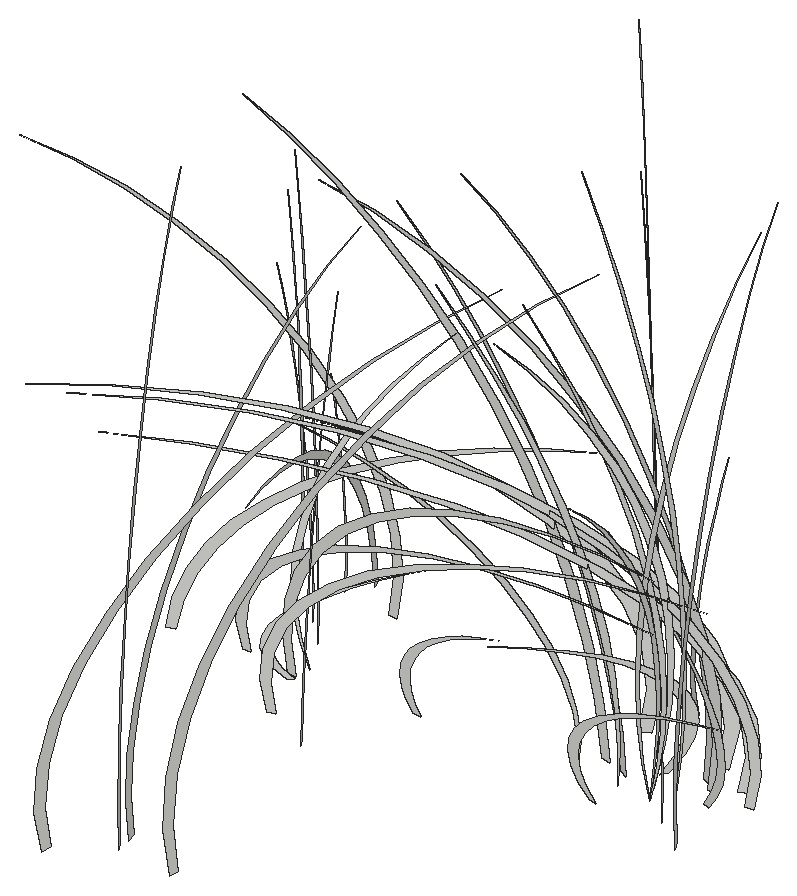
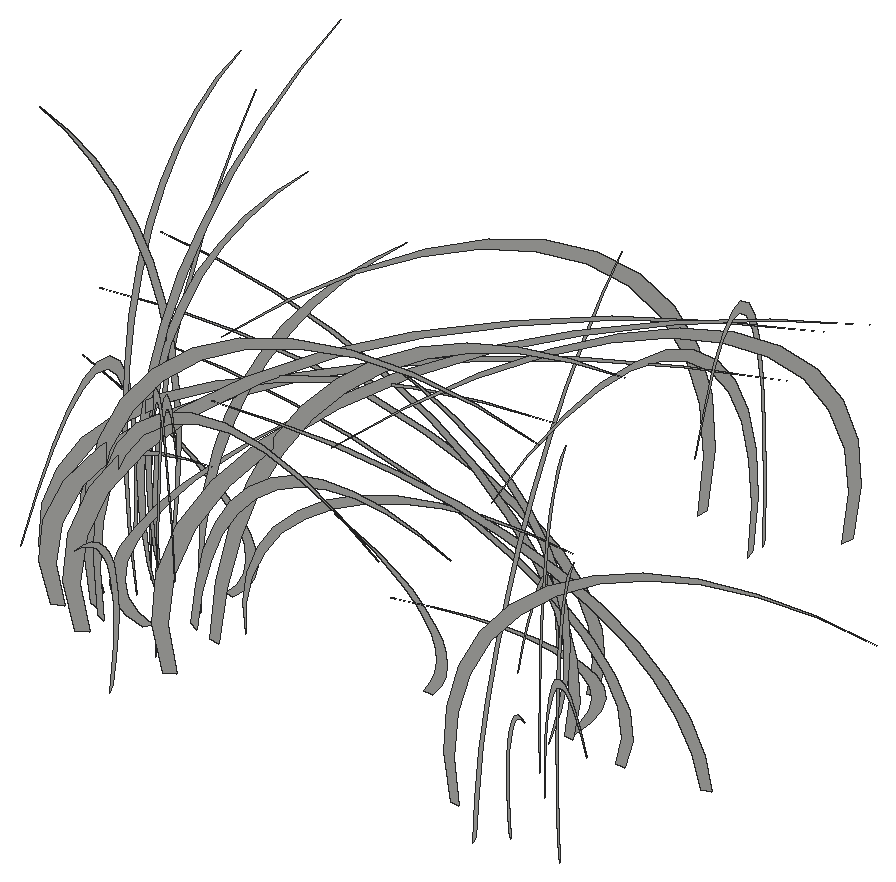
# SketchUp Ruby script. Lengths in inches.
U = 1.inch
M = Sketchup.active_model
def pt(a) = Geom::Point3d.new(a.map { |v| v * U })
def face(e, loops, mat)
  f = e.add_face(loops[0].map { |a| pt(a) })
  loops[1..].each { |l| e.add_face(l.map { |a| pt(a) }).erase! }
  f.material = f.back_material = mat if mat
  f
end
# faces: each face lists its corners as indices into pts; further lists are holes
def faces(e, pts, list, mat = nil) = list.each { |f| face(e, (f[0].is_a?(Array) ? f : [f]).map { |l| l.map { |i| pts[i] } }, mat) }
# xy, xz, yz: faces in a plane at the given z, y or x. An outline is a flat list of corners, or four numbers for a rectangle; further outlines are holes
def ring(l) = l.size == 4 ? [[l[0], l[1]], [l[2], l[1]], [l[2], l[3]], [l[0], l[3]]] : l.each_slice(2).to_a
def flat(e, list, mat, &to3) = list.each { |f| face(e, (f[0].is_a?(Array) ? f : [f]).map { |l| ring(l).map { |u, v| to3.(u, v) } }, mat) }
def xy(e, z, list, mat = nil) = flat(e, list, mat) { |x, y| [x, y, z] }
def xz(e, y, list, mat = nil) = flat(e, list, mat) { |x, z| [x, y, z] }
def yz(e, x, list, mat = nil) = flat(e, list, mat) { |y, z| [x, y, z] }
def lines(e, pts, list) = list.each { |a, b| e.add_line(pt(pts[a]), pt(pts[b])) }
# prism: a flat outline (further loops are holes) pulled along v
def prism(e, loops, v, mat = nil)
  f = face(e, loops, mat); d = Geom::Vector3d.new(v.map { |x| x * U })
  f.pushpull(f.normal.samedirection?(d) ? d.length : -d.length)
end
def box(e, o, s, mat = nil) = prism(e, [[o, [o[0] + s[0], o[1], o[2]], [o[0] + s[0], o[1] + s[1], o[2]], [o[0], o[1] + s[1], o[2]]]], [0, 0, s[2]], mat)
def at(x, y, z, deg = 0) = Geom::Transformation.translation(pt([x, y, z])) * Geom::Transformation.rotation(ORIGIN, Z_AXIS, deg.degrees)
def axes(o, x, y, z) = Geom::Transformation.new([*x, 0, *y, 0, *z, 0, *pt(o).to_a, 1])
def part(name) = M.definitions.add(name)
# library, detail: a bought-in or finely detailed component or shape, given as its bounding box
def library(name, o, s) = part(name).tap { |d| box(d.entities, o, s) }
def detail(e, o, s) = box(e.add_group.entities, o, s)
def put(e, d, t, mat = nil) = e.add_instance(d, t).tap { |i| i.material = mat if mat }
def group(e, t, mat = nil) = e.add_group.tap { |g| g.transformation = t; g.material = mat if mat }.entities
root = M.entities
g1 = group(root,at(18.54,756.38,-58.625))
p = [[-0.31,0.47,0],[-0.14,0.21,0],[0,0,1.44],[-0.06,0.09,2.9],[-0.3,0.46,4.32],[-0.73,1.125,5.68],
  [-1.33,2.05,6.95],[-2.1,3.23,8.08],[-3,4.62,9.06],[-4.02,6.1875,9.85],[-5.13,7.9,10.45],[-6.3,9.71,10.83],
  [-7.52,11.57,10.99],[-8.73,13.45,10.91],[-7.54,11.61,10.93],[-6.36,9.79,10.72],[-5.21,8.03,10.3125],[-4.14,6.37,9.7],
  [-3.15,4.85,8.89],[-2.28,3.51,7.92],[-1.54,2.37,6.8],[-0.95,1.46,5.57],[-0.52,0.8,4.23],[-0.27,0.42,2.84],
  [-0.2,0.31,1.42]]
faces(g1,p,[[0,1,2,3,4,5,6,7,8,9,10,11,12,13,14,15,16,17,18,19,20,21,22,23,24]])
g2 = group(root,at(16.89,755.05,-58.625))
p = [[0.05,0.6,0],[0.02,0.27,0],[0,0,1.23],[0.01,0.11,2.46],[0.05,0.59,3.67],[0.11,1.4375,4.83],
  [0.21,2.62,5.9],[0.32,4.12,6.87],[0.46,5.89,7.7],[0.62,7.89,8.375],[0.79,10.08,8.88],[0.98,12.39,9.21],
  [1.16,14.77,9.34],[1.35,17.16,9.27],[1.17,14.81,9.29],[0.98,12.49,9.12],[0.81,10.25,8.76],[0.64,8.13,8.24],
  [0.49,6.19,7.56],[0.35,4.48,6.73],[0.24,3.02,5.78],[0.15,1.86,4.73],[0.08,1.03,3.6],[0.04,0.53,2.41],
  [0.03,0.39,1.21]]
faces(g2,p,[[0,1,2,3,4,5,6,7,8,9,10,11,12,13,14,15,16,17,18,19,20,21,22,23,24]])
g3 = group(root,at(20.22,756.09,-58.625))
p = [[0.04,0.5625,0],[0.02,0.25,0],[0,0,1.44],[0.01,0.1,2.9],[0.04,0.55,4.32],[0.11,1.34,5.68],
  [0.19,2.44,6.95],[0.3,3.84,8.08],[0.43,5.49,9.06],[0.58,7.35,9.85],[0.74,9.39,10.45],[0.91,11.54,10.83],
  [1.08,13.76,10.99],[1.26,15.99,10.91],[1.09,13.8,10.93],[0.92,11.64,10.72],[0.75,9.55,10.3125],[0.6,7.57,9.7],
  [0.45,5.77,8.89],[0.33,4.17,7.92],[0.22,2.81,6.8],[0.14,1.74,5.57],[0.08,0.96,4.23],[0.04,0.5,2.84],
  [0.03,0.36,1.42]]
faces(g3,p,[[0,1,2,3,4,5,6,7,8,9,10,11,12,13,14,15,16,17,18,19,20,21,22,23,24]])
g4 = group(root,at(18.36,756.9,-58.625))
p = [[-0.16,0.54,0],[-0.07,0.24,0],[0,0,1.26],[-0.03,0.1,2.52],[-0.16,0.53,3.76],[-0.39,1.28,4.94],
  [-0.72,2.34,6.04],[-1.125,3.68,7.03],[-1.61,5.26,7.88],[-2.16,7.05,8.57],[-2.75,9.01,9.09],[-3.38,11.07,9.42],
  [-4.03,13.2,9.56],[-4.6875,15.33,9.49],[-4.05,13.24,9.51],[-3.41,11.16,9.33],[-2.8,9.16,8.97],[-2.22,7.27,8.44],
  [-1.69,5.53,7.74],[-1.22,4,6.89],[-0.83,2.7,5.92],[-0.51,1.66,4.84],[-0.28,0.92,3.68],[-0.15,0.48,2.47],
  [-0.11,0.35,1.23]]
faces(g4,p,[[0,1,2,3,4,5,6,7,8,9,10,11,12,13,14,15,16,17,18,19,20,21,22,23,24]])
g5 = group(root,at(27.14,767.47,-58.625))
p = [[0.12,-0.57,0],[0.05,-0.25,0.92],[0.01,-0.0625,1.85],[0,0,2.78],[0.01,-0.0625,3.71],[0.05,-0.25,4.64],
  [0.12,-0.5625,5.5625],[0.21,-1,6.47],[0.32,-1.55,7.36],[0.46,-2.23,8.23],[0.625,-3.02,9.08],[0.8125,-3.92,9.9],
  [1.02,-4.9375,10.69],[0.82,-3.98,9.89],[0.65,-3.13,9.0625],[0.49,-2.38,8.21],[0.36,-1.74,7.34],[0.25,-1.2,6.45],
  [0.16,-0.77,5.54],[0.09,-0.45,4.625],[0.05,-0.25,3.7],[0.03,-0.16,2.78],[0.04,-0.18,1.85],[0.07,-0.32,0.92]]
faces(g5,p,[[0,1,2,3,4,5,6,7,8,9,10,11,12,13,14,15,16,17,18,19,20,21,22,23]])
g6 = group(root,at(25.3,769.83,-58.625))
p = [[-0.46,-0.32,0],[-0.21,-0.14,0],[0,0,1.26],[-0.08,-0.06,2.52],[-0.45,-0.32,3.76],[-1.1,-0.77,4.94],
  [-2.01,-1.4,6.04],[-3.16,-2.2,7.03],[-4.51,-3.15,7.88],[-6.05,-4.22,8.57],[-7.72,-5.39,9.09],[-9.49,-6.625,9.42],
  [-11.32,-7.9,9.56],[-13.15,-9.17,9.49],[-11.35,-7.92,9.51],[-9.57,-6.68,9.33],[-7.85,-5.48,8.97],[-6.23,-4.35,8.44],
  [-4.75,-3.31,7.74],[-3.43,-2.39,6.89],[-2.32,-1.62,5.92],[-1.43,-1,4.84],[-0.79,-0.55,3.68],[-0.41,-0.28,2.47],
  [-0.3,-0.21,1.23]]
faces(g6,p,[[0,1,2,3,4,5,6,7,8,9,10,11,12,13,14,15,16,17,18,19,20,21,22,23,24]])
g7 = group(root,at(16.66,764.46,-58.625))
p = [[0.46,0.06,0],[0.2,0.03,0],[0,0,0.88],[0.08,0.01,1.76],[0.45,0.06,2.63],[1.1,0.14,3.46],
  [2,0.25,4.23],[3.14,0.4,4.92],[4.5,0.57,5.51],[6.02,0.76,6],[7.69,0.97,6.36],[9.45,1.19,6.59],
  [11.27,1.42,6.6875],[13.09,1.65,6.64],[11.3,1.42,6.65],[9.53,1.2,6.53],[7.82,0.98,6.28],[6.2,0.78,5.9],
  [4.72,0.6,5.41],[3.42,0.43,4.82],[2.31,0.29,4.14],[1.42,0.18,3.39],[0.78,0.1,2.58],[0.41,0.05,1.73],
  [0.3,0.04,0.86]]
faces(g7,p,[[0,1,2,3,4,5,6,7,8,9,10,11,12,13,14,15,16,17,18,19,20,21,22,23,24]])
g8 = group(root,at(29.25,768.92,-58.625))
p = [[-0.55,-0.25,0],[-0.25,-0.11,0],[0,0,1.07],[-0.1,-0.04,2.14],[-0.54,-0.24,3.2],[-1.3125,-0.59,4.2],
  [-2.4,-1.08,5.14],[-3.77,-1.7,5.98],[-5.39,-2.43,6.7],[-7.22,-3.26,7.29],[-9.21,-4.16,7.73],[-11.33,-5.11,8.01],
  [-13.5,-6.1,8.125],[-15.6875,-7.08,8.07],[-13.54,-6.12,8.08],[-11.42,-5.16,7.93],[-9.37,-4.23,7.625],[-7.43,-3.36,7.17],
  [-5.66,-2.56,6.58],[-4.09,-1.85,5.86],[-2.76,-1.25,5.03],[-1.7,-0.77,4.12],[-0.9375,-0.42,3.13],[-0.49,-0.22,2.1],
  [-0.36,-0.16,1.05]]
faces(g8,p,[[0,1,2,3,4,5,6,7,8,9,10,11,12,13,14,15,16,17,18,19,20,21,22,23,24]])
g9 = group(root,at(28.07,769.53,-58.625))
p = [[-0.53,-0.29,0],[-0.24,-0.13,0],[0,0,1.23],[-0.1,-0.05,2.46],[-0.52,-0.28,3.67],[-1.26,-0.69,4.83],
  [-2.31,-1.26,5.9],[-3.625,-1.98,6.87],[-5.18,-2.84,7.7],[-6.95,-3.8,8.375],[-8.87,-4.85,8.88],[-10.9,-5.97,9.21],
  [-13,-7.11,9.34],[-15.1,-8.27,9.27],[-13.03,-7.14,9.29],[-10.99,-6.02,9.12],[-9.02,-4.9375,8.76],[-7.15,-3.92,8.24],
  [-5.45,-2.98,7.56],[-3.9375,-2.16,6.73],[-2.66,-1.46,5.78],[-1.64,-0.9,4.73],[-0.9,-0.49,3.6],[-0.47,-0.26,2.41],
  [-0.34,-0.1875,1.21]]
faces(g9,p,[[0,1,2,3,4,5,6,7,8,9,10,11,12,13,14,15,16,17,18,19,20,21,22,23,24]])
g10 = group(root,at(15.85,766.37,-58.625))
p = [[0.46,-0.05,0],[0.2,-0.02,0],[0,0,1.03],[0.08,-0.01,2.07],[0.45,-0.05,3.09],[1.1,-0.12,4.07],
  [2,-0.22,4.97],[3.15,-0.35,5.79],[4.5,-0.5,6.49],[6.03,-0.67,7.06],[7.7,-0.85,7.48],[9.47,-1.05,7.75],
  [11.29,-1.25,7.87],[13.12,-1.45,7.8125],[11.32,-1.25,7.82],[9.55,-1.05,7.68],[7.83,-0.86,7.38],[6.22,-0.6875,6.94],
  [4.73,-0.52,6.37],[3.42,-0.38,5.67],[2.31,-0.25,4.87],[1.42,-0.16,3.98],[0.78,-0.09,3.03],[0.41,-0.04,2.03],
  [0.3,-0.03,1.02]]
faces(g10,p,[[0,1,2,3,4,5,6,7,8,9,10,11,12,13,14,15,16,17,18,19,20,21,22,23,24]])
g11 = group(root,at(15.85,766.37,-58.625))
p = [[0.46,-0.05,0],[0.2,-0.02,0],[0,0,1.03],[0.08,-0.01,2.07],[0.45,-0.05,3.09],[1.1,-0.12,4.07],
  [2,-0.22,4.97],[3.15,-0.35,5.79],[4.5,-0.5,6.49],[6.03,-0.67,7.06],[7.7,-0.85,7.48],[9.47,-1.05,7.75],
  [11.29,-1.25,7.87],[13.12,-1.45,7.8125],[11.32,-1.25,7.82],[9.55,-1.05,7.68],[7.83,-0.86,7.38],[6.22,-0.6875,6.94],
  [4.73,-0.52,6.37],[3.42,-0.38,5.67],[2.31,-0.25,4.87],[1.42,-0.16,3.98],[0.78,-0.09,3.03],[0.41,-0.04,2.03],
  [0.3,-0.03,1.02]]
faces(g11,p,[[0,1,2,3,4,5,6,7,8,9,10,11,12,13,14,15,16,17,18,19,20,21,22,23,24]])
g12 = group(root,at(25.28,766.12,-58.625))
p = [[5.71,-0.95,4.09],[4.625,-0.77,3.83],[3.64,-0.6,3.54],[2.78,-0.46,3.24],[2.03,-0.34,2.91],[1.41,-0.23,2.57],
  [0.93,-0.15,2.22],[0.59,-0.1,1.85],[0.38,-0.0625,1.48],[0.33,-0.05,1.11],[0.41,-0.07,0.73],[0.64,-0.11,0.36],
  [1.01,-0.17,0],[0.77,-0.125,0],[0.34,-0.06,0.36],[0.07,-0.01,0.73],[-0.04,0.01,1.1],[0.01,0,1.48],
  [0.22,-0.04,1.86],[0.58,-0.1,2.22],[1.1,-0.18,2.58],[1.76,-0.29,2.93],[2.5625,-0.43,3.25],[3.5,-0.58,3.56],
  [4.55,-0.76,3.84]]
faces(g12,p,[[0,1,2,3,4,5,6,7,8,9,10,11,12,13,14,15,16,17,18,19,20,21,22,23,24]])
g13 = group(root,at(27.2,767.97,-58.625))
p = [[-0.25,-0.52,0],[-0.11,-0.23,1.2],[-0.03,-0.06,2.41],[0,0,3.63],[-0.03,-0.06,4.85],[-0.11,-0.23,6.0625],
  [-0.25,-0.52,7.26],[-0.4375,-0.92,8.45],[-0.68,-1.43,9.61],[-0.98,-2.05,10.75],[-1.33,-2.78,11.86],[-1.73,-3.62,12.93],
  [-2.17,-4.55,13.96],[-1.75,-3.67,12.92],[-1.375,-2.89,11.83],[-1.05,-2.19,10.72],[-0.76,-1.6,9.58],[-0.53,-1.1,8.42],
  [-0.34,-0.71,7.24],[-0.2,-0.42,6.04],[-0.11,-0.23,4.84],[-0.07,-0.15,3.625],[-0.08,-0.17,2.41],[-0.14,-0.29,1.2]]
faces(g13,p,[[0,1,2,3,4,5,6,7,8,9,10,11,12,13,14,15,16,17,18,19,20,21,22,23]])
g14 = group(root,at(14.87,771.42,-58.625))
p = [[4.01,-9.63,8.4],[4.61,-11.08,8.62],[4.03,-9.68,8.35],[3.46,-8.32,7.98],[2.92,-7.02,7.51],[2.42,-5.8,6.95],
  [1.95,-4.68,6.3],[1.52,-3.65,5.5625],[1.14,-2.75,4.76],[0.82,-1.97,3.89],[0.55,-1.32,2.97],[0.34,-0.81,2.01],
  [0.19,-0.46,1.02],[0.1,-0.25,0],[0,0,0],[0.07,-0.17,1.04],[0.21,-0.5,2.06],[0.42,-1,3.05],
  [0.6875,-1.65,3.99],[1.02,-2.45,4.87],[1.41,-3.38,5.6875],[1.85,-4.44,6.42],[2.34,-5.61,7.07],[2.86,-6.875,7.62],
  [3.42,-8.22,8.0625]]
faces(g14,p,[[0,1,2,3,4,5,6,7,8,9,10,11,12,13,14,15,16,17,18,19,20,21,22,23,24]])
g15 = group(root,at(14.13,766.64,-58.625))
p = [[0.5,-0.03,0],[0.22,-0.01,0],[0,0,0.75],[0.09,-0.01,1.5],[0.49,-0.03,2.24],[1.18,-0.07,2.94],
  [2.16,-0.13,3.59],[3.39,-0.2,4.18],[4.86,-0.29,4.6875],[6.51,-0.39,5.1],[8.31,-0.5,5.41],[10.21,-0.61,5.6],
  [12.17,-0.73,5.68],[14.14,-0.85,5.64],[12.21,-0.73,5.65],[10.29,-0.62,5.55],[8.44,-0.5,5.33],[6.7,-0.4,5.02],
  [5.1,-0.31,4.6],[3.6875,-0.22,4.1],[2.49,-0.15,3.52],[1.54,-0.09,2.88],[0.85,-0.05,2.19],[0.4375,-0.03,1.47],
  [0.32,-0.02,0.73]]
faces(g15,p,[[0,1,2,3,4,5,6,7,8,9,10,11,12,13,14,15,16,17,18,19,20,21,22,23,24]])
g16 = group(root,at(27.09,769.03,-58.625))
p = [[-2.6,-5.17,4.81],[-2.11,-4.1875,4.5],[-1.66,-3.3,4.17],[-1.26,-2.51,3.81],[-0.92,-1.84,3.43],[-0.64,-1.28,3.02],
  [-0.42,-0.84,2.61],[-0.27,-0.53,2.18],[-0.17,-0.35,1.74],[-0.15,-0.29,1.3],[-0.1875,-0.37,0.86],[-0.29,-0.58,0.43],
  [-0.46,-0.92,0],[-0.35,-0.69,0],[-0.16,-0.31,0.42],[-0.03,-0.07,0.86],[0.02,0.03,1.3],[-0.01,-0.01,1.74],
  [-0.1,-0.2,2.18],[-0.27,-0.53,2.62],[-0.5,-1,3.04],[-0.8,-1.6,3.44],[-1.17,-2.32,3.83],[-1.59,-3.17,4.18],
  [-2.07,-4.12,4.51]]
faces(g16,p,[[0,1,2,3,4,5,6,7,8,9,10,11,12,13,14,15,16,17,18,19,20,21,22,23,24]])
g17 = group(root,at(19.3125,766.77,-58.625))
p = [[3.57,-0.46,3.36],[2.92,-0.375,3.15],[2.33,-0.3,2.92],[1.81,-0.23,2.66],[1.36,-0.17,2.4],[0.99,-0.13,2.12],
  [0.7,-0.09,1.82],[0.49,-0.0625,1.52],[0.37,-0.05,1.22],[0.34,-0.04,0.91],[0.39,-0.05,0.6],[0.53,-0.07,0.3],
  [0.75,-0.1,0],[0.46,-0.06,0],[0.21,-0.03,0.3],[0.06,-0.01,0.61],[0,0,0.93],[0.04,-0.01,1.24],
  [0.17,-0.02,1.55],[0.41,-0.05,1.85],[0.73,-0.09,2.15],[1.14,-0.15,2.43],[1.64,-0.21,2.69],[2.21,-0.28,2.94],
  [2.86,-0.37,3.16]]
faces(g17,p,[[0,1,2,3,4,5,6,7,8,9,10,11,12,13,14,15,16,17,18,19,20,21,22,23,24]])
g18 = group(root,at(27.84,766.85,-58.625))
p = [[-0.58,0.06,0],[-0.26,0.03,1.08],[-0.06,0.01,2.17],[0,0,3.27],[-0.0625,0.01,4.37],[-0.25,0.02,5.46],
  [-0.57,0.06,6.54],[-1.01,0.1,7.61],[-1.58,0.15,8.66],[-2.27,0.22,9.6875],[-3.07,0.3,10.6875],[-3.99,0.39,11.65],
  [-5.02,0.49,12.58],[-4.05,0.4,11.64],[-3.18,0.3125,10.66],[-2.42,0.24,9.66],[-1.76,0.17,8.63],[-1.22,0.12,7.58],
  [-0.78,0.08,6.52],[-0.46,0.05,5.44],[-0.25,0.02,4.36],[-0.16,0.02,3.27],[-0.18,0.02,2.17],[-0.32,0.03,1.08]]
faces(g18,p,[[0,1,2,3,4,5,6,7,8,9,10,11,12,13,14,15,16,17,18,19,20,21,22,23]])
g19 = group(root,at(15.66,765.74,-58.625))
p = [[3.875,2.77,3.36],[3.14,2.25,3.15],[2.47,1.77,2.92],[1.88,1.35,2.66],[1.38,0.99,2.4],[0.96,0.6875,2.12],
  [0.63,0.45,1.82],[0.4,0.28,1.52],[0.26,0.1875,1.22],[0.22,0.16,0.91],[0.28,0.2,0.6],[0.43,0.3125,0.3],
  [0.6875,0.49,0],[0.52,0.37,0],[0.23,0.17,0.3],[0.05,0.04,0.6],[-0.02,-0.02,0.91],[0.01,0.01,1.22],
  [0.15,0.11,1.53],[0.4,0.28,1.83],[0.75,0.53,2.125],[1.2,0.86,2.41],[1.74,1.24,2.68],[2.37,1.7,2.93],
  [3.09,2.21,3.16]]
faces(g19,p,[[0,1,2,3,4,5,6,7,8,9,10,11,12,13,14,15,16,17,18,19,20,21,22,23,24]])
g20 = group(root,at(29.78,768.24,-58.625))
p = [[-0.46,-0.07,0],[-0.2,-0.03,0],[0,0,1.03],[-0.08,-0.01,2.06],[-0.45,-0.07,3.07],[-1.09,-0.18,4.03],
  [-1.98,-0.32,4.93],[-3.11,-0.51,5.74],[-4.45,-0.73,6.43],[-5.97,-0.98,7],[-7.62,-1.25,7.42],[-9.37,-1.53,7.6875],
  [-11.17,-1.83,7.8],[-12.98,-2.125,7.75],[-11.2,-1.83,7.76],[-9.45,-1.55,7.61],[-7.75,-1.27,7.32],[-6.15,-1.01,6.88],
  [-4.68,-0.77,6.3125],[-3.38,-0.55,5.625],[-2.28,-0.375,4.83],[-1.41,-0.23,3.95],[-0.78,-0.13,3.01],[-0.4,-0.07,2.02],
  [-0.29,-0.05,1.01]]
faces(g20,p,[[0,1,2,3,4,5,6,7,8,9,10,11,12,13,14,15,16,17,18,19,20,21,22,23,24]])
g21 = group(root,at(26.22,767.01,-58.625))
p = [[-6.45,0.63,11.96],[-5.42,0.53,11.08],[-4.47,0.4375,10.17],[-3.62,0.35,9.23],[-2.85,0.28,8.26],[-2.17,0.21,7.28],
  [-1.58,0.16,6.27],[-1.09,0.11,5.25],[-0.69,0.07,4.21],[-0.39,0.04,3.17],[-0.19,0.02,2.12],[-0.09,0.01,1.06],
  [-0.08,0.01,0],[0,0,1.0625],[-0.03,0,2.13],[-0.18,0.02,3.19],[-0.4375,0.04,4.25],[-0.8125,0.08,5.29],
  [-1.3,0.13,6.32],[-1.9,0.1875,7.33],[-2.6,0.26,8.32],[-3.41,0.33,9.28],[-4.33,0.42,10.21],[-5.34,0.52,11.1]]
faces(g21,p,[[0,1,2,3,4,5,6,7,8,9,10,11,12,13,14,15,16,17,18,19,20,21,22,23]])
g22 = group(root,at(24.84,767.14,-58.625))
p = [[-10.2,1,6.04],[-8.83,0.87,6],[-7.48,0.73,5.85],[-6.18,0.61,5.6],[-4.95,0.49,5.25],[-3.82,0.375,4.81],
  [-2.81,0.28,4.28],[-1.93,0.1875,3.68],[-1.21,0.12,3.02],[-0.66,0.0625,2.3],[-0.28,0.03,1.55],[-0.09,0.01,0.78],
  [-0.09,0.01,0],[0,0,0.8],[-0.12,0.01,1.59],[-0.45,0.04,2.36],[-0.97,0.1,3.1],[-1.69,0.17,3.79],
  [-2.58,0.25,4.41],[-3.62,0.35,4.94],[-4.79,0.47,5.38],[-6.06,0.59,5.72],[-7.4,0.73,5.94],[-8.79,0.86,6.05]]
faces(g22,p,[[0,1,2,3,4,5,6,7,8,9,10,11,12,13,14,15,16,17,18,19,20,21,22,23]])
g23 = group(root,at(15.98,766.55,-58.625))
p = [[0.38,0.28,0],[0.17,0.13,0.84],[0.04,0.03,1.6875],[0,0,2.54],[0.04,0.03,3.39],[0.17,0.125,4.24],
  [0.38,0.28,5.08],[0.67,0.5,5.91],[1.05,0.78,6.73],[1.5,1.12,7.52],[2.03,1.52,8.3],[2.64,1.97,9.05],
  [3.32,2.48,9.77],[2.68,2,9.04],[2.11,1.58,8.28],[1.6,1.2,7.5],[1.17,0.875,6.7],[0.81,0.6,5.89],
  [0.52,0.39,5.0625],[0.31,0.23,4.23],[0.17,0.125,3.38],[0.11,0.08,2.54],[0.12,0.09,1.6875],[0.21,0.16,0.84]]
faces(g23,p,[[0,1,2,3,4,5,6,7,8,9,10,11,12,13,14,15,16,17,18,19,20,21,22,23]])
g24 = group(root,at(28.3125,767.07,-58.625))
p = [[-0.54,0.2,0],[-0.24,0.09,1.38],[-0.0625,0.02,2.77],[0,0,4.17],[-0.06,0.02,5.57],[-0.24,0.09,6.97],
  [-0.54,0.2,8.35],[-0.96,0.35,9.71],[-1.49,0.54,11.05],[-2.14,0.77,12.36],[-2.9,1.05,13.63],[-3.77,1.36,14.87],
  [-4.74,1.72,16.05],[-3.83,1.38,14.85],[-3.01,1.09,13.6],[-2.29,0.83,12.32],[-1.67,0.6,11.01],[-1.15,0.42,9.68],
  [-0.74,0.27,8.32],[-0.4375,0.16,6.94],[-0.24,0.09,5.56],[-0.15,0.06,4.17],[-0.17,0.0625,2.77],[-0.3,0.11,1.38]]
faces(g24,p,[[0,1,2,3,4,5,6,7,8,9,10,11,12,13,14,15,16,17,18,19,20,21,22,23]])
g25 = group(root,at(12.15,766.27,-58.625))
p = [[9.98,3.05,7.31],[11.48,3.51,7.5],[10.02,3.0625,7.27],[8.61,2.63,6.94],[7.27,2.22,6.54],[6.01,1.84,6.04],
  [4.84,1.48,5.48],[3.79,1.16,4.84],[2.85,0.87,4.14],[2.04,0.62,3.39],[1.37,0.42,2.59],[0.84,0.26,1.75],
  [0.47,0.14,0.88],[0.26,0.08,0],[0,0,0],[0.18,0.05,0.9],[0.52,0.16,1.79],[1.04,0.32,2.65],
  [1.71,0.52,3.47],[2.54,0.78,4.24],[3.5,1.07,4.95],[4.6,1.41,5.59],[5.8125,1.78,6.15],[7.12,2.18,6.63],
  [8.52,2.6,7.02]]
faces(g25,p,[[0,1,2,3,4,5,6,7,8,9,10,11,12,13,14,15,16,17,18,19,20,21,22,23,24]])
g26 = group(root,at(29.36,767.28,-58.625))
p = [[-5.4,2.08,5.53],[-4.375,1.6875,5.18],[-3.45,1.33,4.79],[-2.625,1.01,4.38],[-1.92,0.74,3.9375],[-1.34,0.52,3.48],
  [-0.88,0.34,3],[-0.55,0.21,2.5],[-0.36,0.14,2],[-0.31,0.12,1.5],[-0.39,0.15,0.99],[-0.61,0.23,0.49],
  [-0.96,0.37,0],[-0.72,0.28,0],[-0.32,0.125,0.49],[-0.07,0.03,0.98],[0.03,-0.01,1.49],[-0.01,0,2],
  [-0.21,0.08,2.51],[-0.55,0.21,3.01],[-1.04,0.4,3.49],[-1.67,0.64,3.96],[-2.42,0.9375,4.4],[-3.31,1.28,4.81],
  [-4.3,1.66,5.1875]]
faces(g26,p,[[0,1,2,3,4,5,6,7,8,9,10,11,12,13,14,15,16,17,18,19,20,21,22,23,24]])
g27 = group(root,at(18.62,763.66,-58.625))
p = [[-5.875,8.62,6.21],[-6.76,9.92,6.375],[-5.9,8.66,6.18],[-5.07,7.44,5.9],[-4.28,6.28,5.56],[-3.54,5.19,5.14],
  [-2.85,4.1875,4.66],[-2.23,3.27,4.11],[-1.68,2.46,3.52],[-1.2,1.76,2.88],[-0.81,1.18,2.2],[-0.5,0.73,1.49],
  [-0.28,0.41,0.75],[-0.15,0.22,0],[0,0,0],[-0.1,0.15,0.77],[-0.31,0.45,1.52],[-0.61,0.9,2.25],
  [-1.01,1.48,2.95],[-1.49,2.19,3.6],[-2.0625,3.03,4.21],[-2.71,3.98,4.75],[-3.42,5.02,5.23],[-4.2,6.15,5.63],
  [-5.02,7.36,5.96]]
faces(g27,p,[[0,1,2,3,4,5,6,7,8,9,10,11,12,13,14,15,16,17,18,19,20,21,22,23,24]])
g28 = group(root,at(27.26,766.33,-58.625))
yz(g28,0,[[0.58,0,0.26,1.24,0.06,2.5,0,3.76,0.0625,5.02,0.25,6.28,0.57,7.52,1.02,8.75,1.59,9.96,2.28,11.14,3.08,12.28,4.01,13.39,5.04,14.46,4.07,13.375,3.2,12.25,2.43,11.1,1.77,9.92,1.22,8.72,0.79,7.49,0.46,6.26,0.26,5.01,0.16,3.75,0.1875,2.5,0.32,1.24]])
g29 = group(root,at(25.26,767.8,-58.625))
p = [[-12.4,2.64,12.66],[-14.27,3.03,12.99],[-12.46,2.65,12.59],[-10.71,2.28,12.03],[-9.04,1.92,11.32],[-7.47,1.59,10.47],
  [-6.02,1.28,9.49],[-4.7,1,8.38],[-3.54,0.75,7.17],[-2.53,0.54,5.87],[-1.7,0.36,4.48],[-1.05,0.22,3.03],
  [-0.59,0.125,1.53],[-0.32,0.07,0],[0,0,0],[-0.22,0.05,1.57],[-0.65,0.14,3.1],[-1.29,0.27,4.59],
  [-2.125,0.45,6.01],[-3.15,0.67,7.34],[-4.36,0.93,8.57],[-5.72,1.22,9.68],[-7.22,1.54,10.65],[-8.85,1.88,11.48],
  [-10.58,2.25,12.15]]
faces(g29,p,[[0,1,2,3,4,5,6,7,8,9,10,11,12,13,14,15,16,17,18,19,20,21,22,23,24]])
g30 = group(root,at(28.59,768.16,-58.625))
p = [[-0.55,0.12,0],[-0.25,0.05,0],[0,0,1.44],[-0.1,0.02,2.9],[-0.54,0.11,4.32],[-1.3125,0.28,5.68],
  [-2.4,0.51,6.95],[-3.76,0.8,8.08],[-5.38,1.14,9.06],[-7.22,1.53,9.85],[-9.21,1.96,10.45],[-11.32,2.41,10.83],
  [-13.5,2.87,10.99],[-15.68,3.33,10.91],[-13.54,2.88,10.93],[-11.42,2.43,10.72],[-9.37,1.99,10.3125],[-7.43,1.58,9.7],
  [-5.66,1.2,8.89],[-4.09,0.87,7.92],[-2.76,0.59,6.8],[-1.7,0.36,5.57],[-0.9375,0.2,4.23],[-0.49,0.1,2.84],
  [-0.36,0.08,1.42]]
faces(g30,p,[[0,1,2,3,4,5,6,7,8,9,10,11,12,13,14,15,16,17,18,19,20,21,22,23,24]])
g31 = group(root,at(15.74,767.95,-58.625))
p = [[-3.77,3.77,11.32],[-3.17,3.17,10.48],[-2.62,2.62,9.62],[-2.11,2.11,8.73],[-1.66,1.66,7.82],[-1.27,1.27,6.88],
  [-0.92,0.92,5.93],[-0.64,0.64,4.97],[-0.41,0.41,3.99],[-0.23,0.23,3],[-0.11,0.11,2],[-0.05,0.05,1],
  [-0.05,0.05,0],[0,0,1.01],[-0.02,0.02,2.01],[-0.1,0.1,3.02],[-0.26,0.26,4.02],[-0.48,0.48,5],
  [-0.76,0.76,5.98],[-1.11,1.11,6.93],[-1.52,1.52,7.87],[-2,2,8.78],[-2.53,2.53,9.66],[-3.12,3.12,10.5]]
faces(g31,p,[[0,1,2,3,4,5,6,7,8,9,10,11,12,13,14,15,16,17,18,19,20,21,22,23]])
g32 = group(root,at(16.63,770.23,-58.625))
p = [[-0.46,0.04,0],[-0.21,0.02,0],[0,0,1.1875],[-0.08,0.01,2.38],[-0.45,0.04,3.56],[-1.1,0.09,4.68],
  [-2.01,0.16,5.72],[-3.16,0.25,6.65],[-4.52,0.36,7.45],[-6.05,0.48,8.11],[-7.73,0.61,8.6],[-9.5,0.75,8.91],
  [-11.32,0.89,9.04],[-13.16,1.04,8.98],[-11.36,0.89,8.99],[-9.58,0.75,8.83],[-7.86,0.62,8.49],[-6.23,0.49,7.98],
  [-4.75,0.375,7.32],[-3.43,0.27,6.52],[-2.32,0.18,5.6],[-1.43,0.11,4.58],[-0.79,0.0625,3.48],[-0.41,0.03,2.34],
  [-0.3,0.02,1.17]]
faces(g32,p,[[0,1,2,3,4,5,6,7,8,9,10,11,12,13,14,15,16,17,18,19,20,21,22,23,24]])
g33 = group(root,at(26.02,767.51,-58.625))
p = [[-11.19,5.95,8.88],[-12.88,6.85,9.11],[-11.24,5.98,8.83],[-9.66,5.14,8.4375],[-8.16,4.34,7.94],[-6.74,3.59,7.34],
  [-5.43,2.89,6.66],[-4.25,2.26,5.88],[-3.19,1.7,5.03],[-2.29,1.22,4.12],[-1.53,0.82,3.14],[-0.95,0.5,2.125],
  [-0.53,0.28,1.07],[-0.29,0.16,0],[0,0,0],[-0.2,0.1,1.1],[-0.59,0.3125,2.18],[-1.16,0.62,3.22],
  [-1.92,1.02,4.22],[-2.85,1.51,5.15],[-3.93,2.09,6.01],[-5.16,2.74,6.79],[-6.52,3.47,7.47],[-7.99,4.25,8.05],
  [-9.55,5.08,8.52]]
faces(g33,p,[[0,1,2,3,4,5,6,7,8,9,10,11,12,13,14,15,16,17,18,19,20,21,22,23,24]])
g34 = group(root,at(14.875,770.19,-58.625))
p = [[-2.55,2.55,4.55],[-2.08,2.08,4.26],[-1.66,1.66,3.94],[-1.29,1.29,3.6],[-0.97,0.97,3.24],[-0.71,0.71,2.86],
  [-0.5,0.5,2.47],[-0.35,0.35,2.06],[-0.26,0.26,1.65],[-0.24,0.24,1.23],[-0.28,0.28,0.82],[-0.375,0.375,0.4],
  [-0.53,0.53,0],[-0.33,0.33,0],[-0.15,0.15,0.41],[-0.04,0.04,0.83],[0,0,1.25],[-0.03,0.03,1.68],
  [-0.125,0.125,2.1],[-0.29,0.29,2.51],[-0.52,0.52,2.9],[-0.8125,0.8125,3.28],[-1.17,1.17,3.64],[-1.58,1.58,3.98],
  [-2.04,2.04,4.28]]
faces(g34,p,[[0,1,2,3,4,5,6,7,8,9,10,11,12,13,14,15,16,17,18,19,20,21,22,23,24]])
g35 = group(root,at(13.33,770.36,-58.625))
p = [[-2.55,2.55,9.25],[-2.08,2.08,8.66],[-1.66,1.66,8.02],[-1.29,1.29,7.32],[-0.97,0.97,6.59],[-0.71,0.71,5.81],
  [-0.5,0.5,5.01],[-0.35,0.35,4.1875],[-0.26,0.26,3.35],[-0.24,0.24,2.5],[-0.28,0.28,1.66],[-0.375,0.375,0.82],
  [-0.53,0.53,0],[-0.33,0.33,0],[-0.15,0.15,0.83],[-0.04,0.04,1.68],[0,0,2.54],[-0.03,0.03,3.41],
  [-0.125,0.125,4.26],[-0.29,0.29,5.1],[-0.52,0.52,5.9],[-0.8125,0.8125,6.68],[-1.17,1.17,7.41],[-1.58,1.58,8.08],
  [-2.04,2.04,8.7]]
faces(g35,p,[[0,1,2,3,4,5,6,7,8,9,10,11,12,13,14,15,16,17,18,19,20,21,22,23,24]])
g36 = group(root,at(14.94,768.76,-58.625))
p = [[-5.96,5.96,5.71],[-5.16,5.16,5.67],[-4.37,4.37,5.54],[-3.61,3.61,5.3],[-2.89,2.89,4.97],[-2.23,2.23,4.55],
  [-1.64,1.64,4.05],[-1.13,1.13,3.48],[-0.71,0.71,2.85],[-0.38,0.38,2.18],[-0.16,0.16,1.47],[-0.05,0.05,0.74],
  [-0.05,0.05,0],[0,0,0.75],[-0.07,0.07,1.5],[-0.26,0.26,2.24],[-0.57,0.57,2.9375],[-0.99,0.99,3.58],
  [-1.51,1.51,4.17],[-2.12,2.12,4.67],[-2.8,2.8,5.09],[-3.54,3.54,5.41],[-4.33,4.33,5.62],[-5.14,5.14,5.72]]
faces(g36,p,[[0,1,2,3,4,5,6,7,8,9,10,11,12,13,14,15,16,17,18,19,20,21,22,23]])
g37 = group(root,at(28.1,768.4,-58.625))
p = [[-0.5,0.26,0],[-0.22,0.12,0],[0,0,1.26],[-0.09,0.05,2.52],[-0.49,0.26,3.76],[-1.18,0.63,4.94],
  [-2.16,1.15,6.04],[-3.4,1.81,7.03],[-4.86,2.58,7.88],[-6.51,3.46,8.57],[-8.31,4.42,9.09],[-10.22,5.43,9.42],
  [-12.19,6.48,9.56],[-14.16,7.53,9.49],[-12.22,6.5,9.51],[-10.31,5.48,9.33],[-8.45,4.5,8.97],[-6.71,3.57,8.44],
  [-5.11,2.72,7.74],[-3.69,1.96,6.89],[-2.49,1.33,5.92],[-1.54,0.82,4.84],[-0.85,0.45,3.68],[-0.4375,0.23,2.47],
  [-0.32,0.17,1.23]]
faces(g37,p,[[0,1,2,3,4,5,6,7,8,9,10,11,12,13,14,15,16,17,18,19,20,21,22,23,24]])
g38 = group(root,at(25.87,770.3,-58.625))
p = [[-1.92,3.9375,5.53],[-1.57,3.22,5.18],[-1.25,2.57,4.79],[-0.97,1.99,4.38],[-0.73,1.5,3.9375],[-0.53,1.09,3.48],
  [-0.375,0.77,3],[-0.26,0.54,2.5],[-0.2,0.41,2],[-0.18,0.37,1.5],[-0.21,0.43,0.99],[-0.28,0.58,0.49],
  [-0.4,0.82,0],[-0.25,0.51,0],[-0.11,0.23,0.5],[-0.03,0.0625,1.01],[0,0,1.52],[-0.02,0.04,2.04],
  [-0.09,0.19,2.55],[-0.22,0.45,3.05],[-0.39,0.8,3.53],[-0.61,1.26,3.99],[-0.88,1.8,4.43],[-1.1875,2.4375,4.83],
  [-1.54,3.15,5.2]]
faces(g38,p,[[0,1,2,3,4,5,6,7,8,9,10,11,12,13,14,15,16,17,18,19,20,21,22,23,24]])
g39 = group(root,at(29.45,765.125,-58.625))
p = [[-0.3,0.53,0],[-0.13,0.23,0],[0,0,1.23],[-0.05,0.09,2.46],[-0.3,0.51,3.67],[-0.72,1.25,4.83],
  [-1.3125,2.28,5.9],[-2.06,3.58,6.87],[-2.95,5.125,7.7],[-3.95,6.86,8.375],[-5.04,8.76,8.88],[-6.19,10.77,9.21],
  [-7.39,12.84,9.34],[-8.58,14.92,9.27],[-7.41,12.88,9.29],[-6.25,10.86,9.12],[-5.125,8.91,8.76],[-4.07,7.07,8.24],
  [-3.1,5.38,7.56],[-2.24,3.89,6.73],[-1.51,2.63,5.78],[-0.93,1.62,4.73],[-0.51,0.89,3.6],[-0.27,0.46,2.41],
  [-0.19,0.34,1.21]]
faces(g39,p,[[0,1,2,3,4,5,6,7,8,9,10,11,12,13,14,15,16,17,18,19,20,21,22,23,24]])
g40 = group(root,at(28.36,766.05,-58.625))
p = [[-0.39,0.46,0],[-0.17,0.2,0],[0,0,1.23],[-0.07,0.08,2.46],[-0.39,0.45,3.67],[-0.94,1.1,4.83],
  [-1.71,2,5.9],[-2.68,3.14,6.87],[-3.84,4.49,7.7],[-5.14,6.02,8.375],[-6.57,7.6875,8.88],[-8.07,9.45,9.21],
  [-9.62,11.27,9.34],[-11.18,13.09,9.27],[-9.65,11.3,9.29],[-8.14,9.53,9.12],[-6.68,7.82,8.76],[-5.3,6.2,8.24],
  [-4.03,4.72,7.56],[-2.92,3.41,6.73],[-1.97,2.3,5.78],[-1.21,1.42,4.73],[-0.67,0.78,3.6],[-0.35,0.41,2.41],
  [-0.25,0.3,1.21]]
faces(g40,p,[[0,1,2,3,4,5,6,7,8,9,10,11,12,13,14,15,16,17,18,19,20,21,22,23,24]])
g41 = group(root,at(25.89,768.94,-58.625))
p = [[-8.23,9.64,12.66],[-9.47,11.09,12.99],[-8.27,9.68,12.59],[-7.11,8.32,12.03],[-6,7.03,11.32],[-4.96,5.81,10.47],
  [-4,4.68,9.49],[-3.125,3.66,8.38],[-2.35,2.75,7.17],[-1.68,1.97,5.87],[-1.13,1.32,4.48],[-0.7,0.82,3.03],
  [-0.39,0.46,1.53],[-0.21,0.25,0],[0,0,0],[-0.14,0.17,1.57],[-0.43,0.51,3.1],[-0.86,1,4.59],
  [-1.41,1.65,6.01],[-2.09,2.45,7.34],[-2.89,3.39,8.57],[-3.8,4.45,9.68],[-4.8,5.62,10.65],[-5.88,6.88,11.48],
  [-7.03,8.23,12.15]]
faces(g41,p,[[0,1,2,3,4,5,6,7,8,9,10,11,12,13,14,15,16,17,18,19,20,21,22,23,24]])
